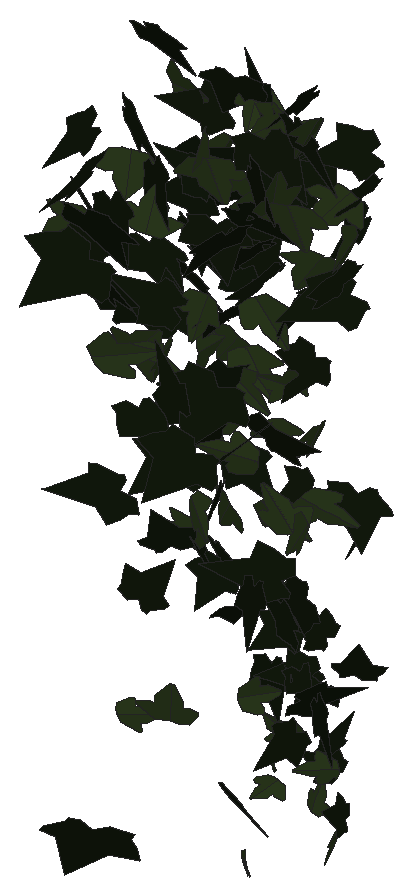
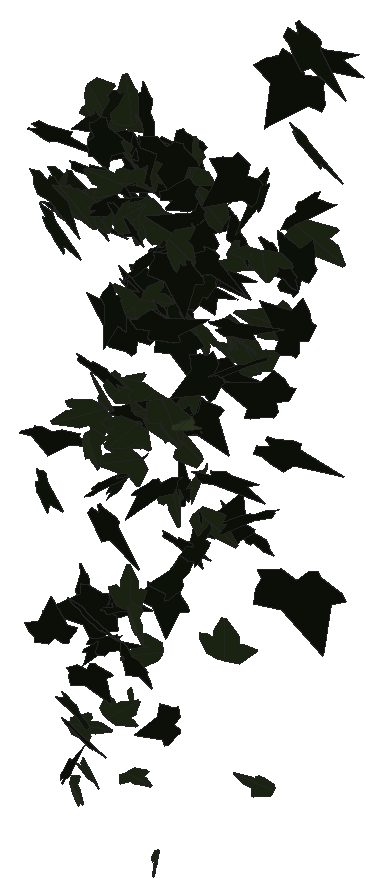
# SketchUp Ruby script. Lengths in inches.
U = 1.inch
M = Sketchup.active_model
def pt(a) = Geom::Point3d.new(a.map { |v| v * U })
def face(e, loops, mat)
  f = e.add_face(loops[0].map { |a| pt(a) })
  loops[1..].each { |l| e.add_face(l.map { |a| pt(a) }).erase! }
  f.material = f.back_material = mat if mat
  f
end
# faces: each face lists its corners as indices into pts; further lists are holes
def faces(e, pts, list, mat = nil) = list.each { |f| face(e, (f[0].is_a?(Array) ? f : [f]).map { |l| l.map { |i| pts[i] } }, mat) }
# xy, xz, yz: faces in a plane at the given z, y or x. An outline is a flat list of corners, or four numbers for a rectangle; further outlines are holes
def ring(l) = l.size == 4 ? [[l[0], l[1]], [l[2], l[1]], [l[2], l[3]], [l[0], l[3]]] : l.each_slice(2).to_a
def flat(e, list, mat, &to3) = list.each { |f| face(e, (f[0].is_a?(Array) ? f : [f]).map { |l| ring(l).map { |u, v| to3.(u, v) } }, mat) }
def xy(e, z, list, mat = nil) = flat(e, list, mat) { |x, y| [x, y, z] }
def xz(e, y, list, mat = nil) = flat(e, list, mat) { |x, z| [x, y, z] }
def yz(e, x, list, mat = nil) = flat(e, list, mat) { |y, z| [x, y, z] }
def lines(e, pts, list) = list.each { |a, b| e.add_line(pt(pts[a]), pt(pts[b])) }
# prism: a flat outline (further loops are holes) pulled along v
def prism(e, loops, v, mat = nil)
  f = face(e, loops, mat); d = Geom::Vector3d.new(v.map { |x| x * U })
  f.pushpull(f.normal.samedirection?(d) ? d.length : -d.length)
end
def box(e, o, s, mat = nil) = prism(e, [[o, [o[0] + s[0], o[1], o[2]], [o[0] + s[0], o[1] + s[1], o[2]], [o[0], o[1] + s[1], o[2]]]], [0, 0, s[2]], mat)
def at(x, y, z, deg = 0) = Geom::Transformation.translation(pt([x, y, z])) * Geom::Transformation.rotation(ORIGIN, Z_AXIS, deg.degrees)
def axes(o, x, y, z) = Geom::Transformation.new([*x, 0, *y, 0, *z, 0, *pt(o).to_a, 1])
def part(name) = M.definitions.add(name)
# library, detail: a bought-in or finely detailed component or shape, given as its bounding box
def library(name, o, s) = part(name).tap { |d| box(d.entities, o, s) }
def detail(e, o, s) = box(e.add_group.entities, o, s)
def put(e, d, t, mat = nil) = e.add_instance(d, t).tap { |i| i.material = mat if mat }
def group(e, t, mat = nil) = e.add_group.tap { |g| g.transformation = t; g.material = mat if mat }.entities
root = M.entities
M.materials.add("1026 AP 7946 SUNNY SIDE UP").color = [254, 231, 186]
M.materials.add("efeu1").color = [18, 25, 13]
M.materials.add("efeu2").color = [43, 57, 29]
c1 = part("ivyleaf_9")
p = [[1.54,2.16,1.25],[1.36,2.04,1.19],[-0.21,0.99,0.68],[-0.71,1.11,0.82],[-0.85,0.86,0.67],[-0.8,0.17,0.21],
  [-0.9,-0.01,0.1],[-0.67,-0.16,-0.02],[-0.08,-0.08,-0.05],[-0.03,-0.6,-0.4],[0.65,-0.88,-0.66],[0.83,-0.6,-0.49],
  [1.29,-0.42,-0.43],[1.8125,-0.07,-0.26],[1.21,0.44,0.15]]
faces(c1.entities,p,[[0,1,2,3,4,5,6,7,8,9,10,11,12,13,14]],"efeu1")
c2 = part("ivyleaf_10")
p = [[0,0.5,-0.03],[-0.0625,2.02,-0.43],[-0.19,2.01,-0.46],[-0.54,1.05,-0.29],[-0.52,0.625,-0.18],[-0.83,0.76,-0.28],
  [-1.16,0.64,-0.33],[-1.15,0.33,-0.24],[-0.77,-0.39,0.02],[-0.3,-0.51,0.16],[0.04,-0.48,0.23],[-0.02,2.01,-0.4375],
  [-0.06,2.01,-0.43],[0.04,-0.49,0.23],[0.67,-0.49,0.14],[1.38,0.36,-0.2],[1.375,0.51,-0.24],[0.81,0.65,-0.19],
  [0.62,0.59,-0.15],[0.6,1.09,-0.28],[0.5,1.23,-0.31]]
faces(c2.entities,p,[[0,1,2,3,4,5,6,7,8,9,10],[11,12,0,13,14,15,16,17,18,19,20]],"efeu2")
put(root,c1,axes([142.13,203.52,266.92],[-0.59838,-0.25995,0.14465],[-0.15209,-0.10927,-0.47412],[0.44014,-0.39117,0.03283]),"1026 AP 7946 SUNNY SIDE UP")
put(root,c1,axes([142.22,203.6,254.35],[0.33655,0.29324,-0.32482],[-0.26346,-0.26965,-0.37513],[-0.62578,0.27124,-0.01675]),"1026 AP 7946 SUNNY SIDE UP")
put(root,c1,axes([141.34,204.61,268.11],[-0.41422,0.33967,-0.1751],[0.1295,-0.15324,-0.44287],[-0.58443,-0.27471,0.02597]),"1026 AP 7946 SUNNY SIDE UP")
put(root,c1,axes([141.35,204.56,267.15],[0.68349,0.0532,-0.11463],[-0.16482,-0.05756,-0.4493],[-0.10301,0.44506,-0.04172]),"1026 AP 7946 SUNNY SIDE UP")
put(root,c1,axes([143.26,205.375,262.24],[-0.60942,-0.18272,0.00796],[0.01229,-0.03707,-0.44],[0.28737,-0.3859,0.03571]),"1026 AP 7946 SUNNY SIDE UP")
put(root,c1,axes([144.04,206.29,259.13],[-0.33232,0.03705,-0.34007],[0.49382,-0.10596,-0.21987],[-0.17119,-0.37756,0.02593]),"1026 AP 7946 SUNNY SIDE UP")
put(root,c1,axes([139.9,206.48,265.28],[0.05679,-0.12956,-0.36457],[0.20893,-0.3275,0.13586],[-0.55334,-0.13696,0.01388]),"1026 AP 7946 SUNNY SIDE UP")
put(root,c1,axes([142.28,206.16,262.59],[-0.1674,-0.29108,0.27585],[0.11646,0.25946,0.32045],[-0.61269,0.12885,-0.01446]),"1026 AP 7946 SUNNY SIDE UP")
put(root,c1,axes([143.36,206.1,261.8],[-0.12627,0.36421,-0.14879],[-0.03686,0.14481,0.38499],[0.61618,0.0833,-0.00746]),"1026 AP 7946 SUNNY SIDE UP")
put(root,c1,axes([142.68,206.83,262.8],[-0.60903,-0.22483,-0.08626],[0.14251,0.00751,-0.45963],[0.34854,-0.39594,0.0372]),"1026 AP 7946 SUNNY SIDE UP")
put(root,c1,axes([140.22,206.88,259.71],[-0.09943,-0.11542,-0.35875],[-0.37918,-0.25236,0.13005],[-0.43344,0.24724,-0.03147]),"1026 AP 7946 SUNNY SIDE UP")
put(root,c1,axes([144.11,206.95,259.09],[-0.30554,-0.0104,0.33923],[-0.50482,-0.08012,-0.19822],[0.11666,-0.37391,0.03075]),"1026 AP 7946 SUNNY SIDE UP")
put(root,c1,axes([139.48,206.94,267.4],[-0.51522,0.16645,-0.14793],[0.16639,-0.10839,-0.37636],[-0.30408,-0.34133,0.0447]),"1026 AP 7946 SUNNY SIDE UP")
put(root,c2,axes([139.25,207.05,265.23],[-0.35022,-0.11625,0.30223],[-0.35381,-0.19439,-0.25591],[0.34927,-0.31349,0.04382]),"1026 AP 7946 SUNNY SIDE UP")
put(root,c2,axes([140.03,206.78,262.63],[-0.15968,-0.07963,0.36959],[0.3595,0.2783,0.13178],[-0.45328,0.24878,-0.02569]),"1026 AP 7946 SUNNY SIDE UP")
put(root,c1,axes([142.73,207.02,266.11],[-0.15301,0.33929,-0.26201],[0.07773,-0.25207,-0.36464],[-0.66403,-0.10769,0.01768]),"1026 AP 7946 SUNNY SIDE UP")
put(root,c1,axes([140.64,207.07,257.44],[-0.27102,0.20408,0.21536],[0.24627,-0.13876,0.27329],[0.38624,0.23168,-0.02313]),"1026 AP 7946 SUNNY SIDE UP")
put(root,c2,axes([141.07,207.46,254.83],[-0.50153,-0.12449,-0.00868],[-0.02899,0.02609,0.35143],[-0.19397,0.31798,-0.03007]),"1026 AP 7946 SUNNY SIDE UP")
put(root,c1,axes([143.97,207.52,257.72],[0.01058,-0.34074,0.11709],[0.00193,0.11563,0.35176],[-0.56577,-0.00598,0.00339]),"1026 AP 7946 SUNNY SIDE UP")
put(root,c2,axes([143.51,207.62,266.85],[-0.14274,-0.37927,-0.07801],[-0.0417,-0.06928,0.40123],[-0.60604,0.09409,-0.00923]),"1026 AP 7946 SUNNY SIDE UP")
put(root,c1,axes([143.3,207.67,261.59],[0.06292,-0.11241,0.37205],[0.44095,-0.23581,-0.10882],[0.40052,0.27728,0.06135]),"1026 AP 7946 SUNNY SIDE UP")
put(root,c2,axes([140.82,207.61,262.67],[0.12967,-0.3648,-0.01894],[-0.01585,0.01445,-0.38515],[0.57397,0.08281,-0.00635]),"1026 AP 7946 SUNNY SIDE UP")
put(root,c1,axes([143.78,207.85,255.18],[-0.01763,-0.03729,-0.36455],[0.20536,-0.32953,0.0296],[-0.52009,-0.12885,0.02405]),"1026 AP 7946 SUNNY SIDE UP")
put(root,c1,axes([142.82,207.79,267.21],[0.06414,-0.06484,-0.39952],[0.59443,-0.09942,0.05756],[-0.16793,-0.37669,0.05115]),"1026 AP 7946 SUNNY SIDE UP")
put(root,c2,axes([143.94,207.61,266.78],[-0.57044,-0.11345,-0.0675],[0.11788,-0.02386,-0.38903],[0.16833,-0.36776,0.0437]),"1026 AP 7946 SUNNY SIDE UP")
put(root,c1,axes([138.63,208.02,264.84],[0.07673,-0.20187,0.41712],[0.18726,-0.38834,-0.21592],[0.68798,0.12822,0.01225]),"1026 AP 7946 SUNNY SIDE UP")
put(root,c2,axes([140.13,207.8,262.27],[-0.05549,-0.01653,-0.3496],[0.4883,-0.13976,-0.02708],[-0.21638,-0.31115,0.02855]),"1026 AP 7946 SUNNY SIDE UP")
put(root,c1,axes([143.13,207.6875,264.95],[-0.24728,0.38585,-0.01038],[-0.01578,-0.01733,-0.42904],[-0.60682,-0.15679,0.01539]),"1026 AP 7946 SUNNY SIDE UP")
put(root,c2,axes([139.96,207.85,262.29],[-0.47982,-0.06192,0.15725],[0.22931,0.04941,0.32055],[-0.12152,0.33776,-0.01598]),"1026 AP 7946 SUNNY SIDE UP")
put(root,c1,axes([138.6,208.12,263.45],[0.20155,-0.20763,0.37149],[0.25656,-0.32337,-0.25263],[0.60364,0.20677,-0.01666]),"1026 AP 7946 SUNNY SIDE UP")
put(root,c1,axes([139.13,208.07,265.125],[-0.23987,-0.03836,-0.3583],[0.5497,-0.00751,-0.15725],[0.01336,-0.37951,0.03709]),"1026 AP 7946 SUNNY SIDE UP")
put(root,c2,axes([143.88,207.95,259.69],[0.29643,-0.30327,-0.08176],[-0.07717,0.06088,-0.36739],[0.48616,0.19458,-0.00846]),"1026 AP 7946 SUNNY SIDE UP")
put(root,c1,axes([140.55,208.09,258.125],[0.28484,0.08872,0.25547],[-0.37665,-0.06815,0.2054],[0.17036,-0.29902,0.02699]),"1026 AP 7946 SUNNY SIDE UP")
put(root,c2,axes([141.25,208.01,259.23],[-0.0883,0.33883,0.04532],[-0.02443,0.04005,-0.35348],[-0.53632,-0.05761,0.00864]),"1026 AP 7946 SUNNY SIDE UP")
put(root,c1,axes([144.01,208.32,255.64],[-0.08166,-0.01533,-0.39435],[0.5788,-0.10871,-0.04761],[-0.1664,-0.3706,0.02792]),"1026 AP 7946 SUNNY SIDE UP")
put(root,c1,axes([141.25,208.21,260.82],[-0.05853,0.23373,-0.25671],[0.02904,-0.25025,-0.24483],[-0.53794,-0.03894,0.01472]),"1026 AP 7946 SUNNY SIDE UP")
put(root,c1,axes([141.89,208.17,253.11],[0.39149,-0.16311,0.04338],[0.03946,-0.04005,-0.30621],[0.2623,0.24947,-0.01868]),"1026 AP 7946 SUNNY SIDE UP")
put(root,c1,axes([142.41,208.04,266.1],[0.54405,0.09283,0.09657],[0.15538,-0.01027,-0.36741],[-0.13654,0.35818,-0.03332]),"1026 AP 7946 SUNNY SIDE UP")
put(root,c2,axes([143.37,208.1875,259.53],[0.44804,0.07573,0.20431],[-0.31486,-0.01218,0.30176],[0.10892,-0.3467,0.0319]),"1026 AP 7946 SUNNY SIDE UP")
put(root,c1,axes([140.37,208.33,263.17],[-0.32606,-0.20416,-0.17098],[-0.21293,-0.09665,0.29831],[-0.35338,0.24662,-0.02198]),"1026 AP 7946 SUNNY SIDE UP")
put(root,c2,axes([141.09,208.46,267.04],[-0.06813,0.16566,-0.30754],[-0.01053,-0.30221,-0.173],[-0.53803,-0.01506,0.04233]),"1026 AP 7946 SUNNY SIDE UP")
put(root,c1,axes([141.51,208.44,257.74],[-0.45217,-0.04754,-0.10807],[0.16951,-0.01388,-0.29881],[0.06262,-0.30569,0.02854]),"1026 AP 7946 SUNNY SIDE UP")
put(root,c2,axes([140.91,208.35,258.43],[-0.24914,-0.0192,0.27815],[-0.4065,-0.08239,-0.16275],[0.12668,-0.30212,0.0248]),"1026 AP 7946 SUNNY SIDE UP")
put(root,c2,axes([142.13,208.44,260.41],[0.0036,0.03782,0.3531],[-0.48914,-0.14717,0.01802],[0.23317,-0.30931,0.03235]),"1026 AP 7946 SUNNY SIDE UP")
put(root,c1,axes([144.61,208.25,265.18],[-0.30351,0.37172,0.0393],[-0.07983,0.01407,-0.42959],[-0.58179,-0.19585,0.03845]),"1026 AP 7946 SUNNY SIDE UP")
put(root,c2,axes([139.84,208.29,264.83],[0.44649,0.1982,-0.10615],[0.09931,0.0905,0.35529],[0.33777,-0.2886,0.03585]),"1026 AP 7946 SUNNY SIDE UP")
put(root,c1,axes([140.42,208.61,259.73],[-0.56399,-0.13094,0.05247],[-0.05681,-0.0511,-0.39198],[0.21394,-0.35877,0.03426]),"1026 AP 7946 SUNNY SIDE UP")
put(root,c1,axes([144.47,208.61,264.73],[-0.63382,-0.03907,0.09414],[-0.13126,-0.07575,-0.41212],[0.08541,-0.40637,0.06529]),"1026 AP 7946 SUNNY SIDE UP")
put(root,c2,axes([141.28,208.43,266.53],[-0.54369,-0.18316,-0.08286],[0.14254,-0.00259,-0.40058],[0.27966,-0.35476,0.04308]),"1026 AP 7946 SUNNY SIDE UP")
put(root,c1,axes([141.27,208.53,258.97],[0.03668,0.20271,0.24666],[-0.12288,-0.22759,0.20601],[0.47631,-0.07432,0.03415]),"1026 AP 7946 SUNNY SIDE UP")
put(root,c1,axes([139.71,208.66,265.8125],[-0.14746,-0.01813,-0.38421],[0.57634,-0.0773,-0.09156],[-0.11119,-0.37661,0.03499]),"1026 AP 7946 SUNNY SIDE UP")
put(root,c2,axes([143.77,208.4375,260.01],[-0.25443,-0.11091,-0.30979],[0.45648,0.0904,-0.19516],[0.21138,-0.32872,0.04857]),"1026 AP 7946 SUNNY SIDE UP")
put(root,c1,axes([139.24,208.46,266.98],[0.41531,-0.21474,-0.24183],[-0.30938,0.12749,-0.34929],[0.39132,0.3287,-0.01949]),"1026 AP 7946 SUNNY SIDE UP")
put(root,c2,axes([143.73,208.65,265.2],[-0.38701,-0.21539,0.15319],[-0.14334,-0.12258,-0.3363],[0.38695,-0.26083,0.02864]),"1026 AP 7946 SUNNY SIDE UP")
put(root,c2,axes([140.85,208.69,263.24],[0.52504,-0.16914,0.03698],[0.03354,-0.03927,-0.38495],[0.27012,0.33363,-0.02409]),"1026 AP 7946 SUNNY SIDE UP")
put(root,c1,axes([140.6875,208.64,258.12],[0.43114,-0.24511,-0.09537],[-0.13525,0.04024,-0.37766],[0.38834,0.28614,-0.02565]),"1026 AP 7946 SUNNY SIDE UP")
put(root,c2,axes([142.6,208.66,259.38],[-0.32619,0.01013,-0.28697],[0.42819,-0.06712,-0.21178],[-0.09402,-0.34082,0.0311]),"1026 AP 7946 SUNNY SIDE UP")
put(root,c1,axes([143.45,208.59,257.71],[0.024,-0.02601,-0.38442],[-0.58645,-0.0276,-0.0139],[-0.04181,0.37229,-0.02568]),"1026 AP 7946 SUNNY SIDE UP")
put(root,c2,axes([141.57,208.66,259.02],[-0.36426,0.14355,0.20412],[-0.29439,0.06994,-0.27844],[-0.24608,-0.29616,0.03095]),"1026 AP 7946 SUNNY SIDE UP")
put(root,c1,axes([142.63,209.07,266.1],[-0.22773,-0.21111,0.28057],[-0.18168,-0.24994,-0.2632],[0.51205,-0.18257,0.03139]),"1026 AP 7946 SUNNY SIDE UP")
put(root,c1,axes([141.08,208.86,264.93],[-0.27977,-0.23134,-0.19605],[0.22292,0.12823,-0.29845],[0.41344,-0.22568,0.02826]),"1026 AP 7946 SUNNY SIDE UP")
put(root,c2,axes([143.4,208.89,267.96],[-0.01035,-0.33417,0.11126],[-0.00626,-0.10984,-0.34497],[0.5531,-0.0075,-0.00182]),"1026 AP 7946 SUNNY SIDE UP")
put(root,c1,axes([140.6,208.97,265.82],[-0.04066,-0.34119,-0.01525],[-0.00547,-0.01264,0.35241],[-0.53683,0.02597,-0.00243]),"1026 AP 7946 SUNNY SIDE UP")
put(root,c2,axes([138.91,208.88,265.65],[0.54423,0.13229,-0.00426],[0.01062,-0.03132,-0.38051],[-0.20789,0.34473,-0.0306]),"1026 AP 7946 SUNNY SIDE UP")
put(root,c1,axes([142.29,208.86,267.22],[-0.1201,-0.25737,-0.29935],[0.26288,0.24385,-0.26771],[0.54895,-0.17308,0.06271]),"1026 AP 7946 SUNNY SIDE UP")
put(root,c1,axes([140.32,209.15,264.31],[0.03429,-0.2502,0.28769],[0.05261,-0.27874,-0.26028],[0.58888,0.03947,0.0065]),"1026 AP 7946 SUNNY SIDE UP")
put(root,c1,axes([143.4375,208.58,255.49],[0.04481,0.24141,-0.29325],[-0.00017,0.28686,0.25109],[0.58852,-0.0183,0.0224]),"1026 AP 7946 SUNNY SIDE UP")
put(root,c2,axes([142.01,208.67,255.01],[-0.00973,-0.00463,0.32185],[0.07578,0.30875,0.0075],[-0.48546,0.04829,-0.00528]),"1026 AP 7946 SUNNY SIDE UP")
put(root,c1,axes([142.91,209.03,267.69],[0.35432,-0.36658,0.01932],[-0.00764,-0.02742,-0.44304],[0.57729,0.22463,-0.01772]),"1026 AP 7946 SUNNY SIDE UP")
put(root,c1,axes([140.09,208.87,262.4],[-0.55136,-0.01566,0.07396],[0.10995,0.03782,0.36012],[-0.03593,0.35594,-0.0329]),"1026 AP 7946 SUNNY SIDE UP")
put(root,c2,axes([142.01,209.02,263.42],[0.42972,0.04242,0.2566],[0.39137,0.01583,-0.2843],[-0.06614,0.36927,-0.0151]),"1026 AP 7946 SUNNY SIDE UP")
put(root,c2,axes([140.625,209.11,260.43],[0.22366,-0.11455,-0.33538],[0.44381,-0.16279,0.18548],[-0.3106,-0.31511,0.02352]),"1026 AP 7946 SUNNY SIDE UP")
put(root,c1,axes([141.14,208.95,263.01],[-0.01218,0.32028,-0.11176],[0.00391,-0.11027,-0.33069],[-0.53262,-0.00813,0.00013]),"1026 AP 7946 SUNNY SIDE UP")
put(root,c2,axes([142.45,208.86,253.8],[-0.04774,0.08133,0.28033],[-0.2767,0.20883,-0.08345],[-0.34963,-0.17637,0.02776]),"1026 AP 7946 SUNNY SIDE UP")
put(root,c1,axes([141.45,208.92,256.6875],[0.12001,0.2845,-0.0232],[0.00137,-0.02522,-0.30351],[-0.44896,0.07597,-0.00713]),"1026 AP 7946 SUNNY SIDE UP")
put(root,c2,axes([143.96,209.35,265.41],[0.06003,-0.08873,0.38543],[0.22311,-0.34674,-0.10153],[0.56277,0.14693,-0.00087]),"1026 AP 7946 SUNNY SIDE UP")
put(root,c2,axes([142.01,209.12,265.79],[-0.29896,-0.31855,-0.03717],[0.05925,0.01734,-0.38131],[0.50028,-0.19241,0.02295]),"1026 AP 7946 SUNNY SIDE UP")
put(root,c1,axes([138.62,208.91,262.27],[-0.00831,0.03444,0.39447],[0.5491,0.16014,-0.00894],[-0.25213,0.34764,-0.03248]),"1026 AP 7946 SUNNY SIDE UP")
put(root,c1,axes([140.42,209.18,265.33],[-0.01987,-0.04755,-0.36037],[-0.52241,-0.11593,0.02794],[-0.1864,0.32999,-0.0399]),"1026 AP 7946 SUNNY SIDE UP")
put(root,c1,axes([142.39,209.4375,256.31],[-0.29398,-0.15325,0.14812],[-0.14848,-0.11195,-0.24858],[0.29624,-0.2082,0.0224]),"1026 AP 7946 SUNNY SIDE UP")
put(root,c2,axes([138.59,209.2,253.22],[0.12049,-0.02499,-0.23886],[0.36578,0.02315,0.07681],[0.02246,-0.24296,0.03044]),"1026 AP 7946 SUNNY SIDE UP")
put(root,c1,axes([140.71,209.39,257.52],[0.31388,-0.27413,0.07524],[0.04444,-0.07156,-0.34923],[0.4445,0.20073,-0.01822]),"1026 AP 7946 SUNNY SIDE UP")
put(root,c1,axes([140.83,209.08,261.27],[0.05366,0.03754,0.34863],[0.44855,0.18215,-0.04941],[-0.2917,0.287,-0.01186]),"1026 AP 7946 SUNNY SIDE UP")
put(root,c1,axes([144.09,209.42,259.84],[-0.30108,-0.25414,-0.15768],[0.18671,0.09943,-0.3256],[0.42622,-0.22308,0.03125]),"1026 AP 7946 SUNNY SIDE UP")
put(root,c1,axes([140.12,209.13,265.87],[0.1257,0.04792,0.3873],[0.55013,0.13766,-0.09398],[-0.228,0.35857,-0.01324]),"1026 AP 7946 SUNNY SIDE UP")
put(root,c2,axes([140.52,209.1,261.96],[0.02725,-0.0465,-0.34816],[0.11097,0.33129,-0.04133],[0.52439,-0.06769,0.02684]),"1026 AP 7946 SUNNY SIDE UP")
put(root,c2,axes([141.17,209.42,265.83],[-0.3904,-0.07011,0.2606],[-0.3618,-0.11058,-0.26446],[0.19991,-0.33706,0.03029]),"1026 AP 7946 SUNNY SIDE UP")
put(root,c1,axes([141.9,209.51,255.29],[-0.2843,-0.03128,-0.30027],[0.46063,-0.01503,-0.18575],[0.00575,-0.34252,0.03355]),"1026 AP 7946 SUNNY SIDE UP")
put(root,c2,axes([142.25,209.58,261.55],[-0.13496,-0.11238,-0.27387],[-0.26605,-0.20427,0.14439],[-0.36652,0.18966,-0.00397]),"1026 AP 7946 SUNNY SIDE UP")
put(root,c1,axes([141.54,209.29,264.43],[0.03195,0.32467,-0.07917],[-0.00744,-0.07855,-0.33559],[-0.52524,0.02086,-0.00006]),"1026 AP 7946 SUNNY SIDE UP")
put(root,c2,axes([141.08,209.46,261.3],[0.23695,0.02622,0.31429],[0.48122,-0.01565,-0.15452],[0.00389,0.33977,-0.02937]),"1026 AP 7946 SUNNY SIDE UP")
put(root,c2,axes([142.03,209.39,260.65],[-0.42066,-0.06566,-0.16391],[0.25354,0.00529,-0.28219],[0.09312,-0.31103,0.0279]),"1026 AP 7946 SUNNY SIDE UP")
put(root,c1,axes([142.62,209.17,263.43],[-0.0713,0.0014,-0.40462],[-0.42762,0.28516,0.03506],[0.44561,0.27388,-0.0311]),"1026 AP 7946 SUNNY SIDE UP")
put(root,c1,axes([138.7,209.49,259.79],[0.07226,-0.32268,-0.16969],[0.09011,0.16862,-0.32649],[0.56117,0.01447,0.07427]),"1026 AP 7946 SUNNY SIDE UP")
put(root,c1,axes([142.74,209.64,255.33],[-0.26659,-0.06096,0.23447],[-0.31379,-0.11272,-0.18463],[0.19796,-0.26077,0.02311]),"1026 AP 7946 SUNNY SIDE UP")
put(root,c1,axes([142.64,209.51,255.38],[0.05084,-0.23142,-0.15291],[-0.0251,0.14629,-0.23983],[0.43045,0.03586,0.00408]),"1026 AP 7946 SUNNY SIDE UP")
put(root,c1,axes([141.54,209.8,264.84],[-0.16019,-0.14956,0.31096],[-0.23244,-0.2645,-0.18743],[0.4773,-0.17901,0.01309]),"1026 AP 7946 SUNNY SIDE UP")
put(root,c2,axes([142.03,209.5,267.34],[0.34347,-0.21334,-0.18901],[-0.24398,0.10061,-0.31231],[0.36762,0.2661,-0.03068]),"1026 AP 7946 SUNNY SIDE UP")
put(root,c1,axes([142.8,209.72,266.71],[-0.59173,-0.10881,-0.03608],[0.07117,-0.0335,-0.40114],[0.16473,-0.3764,0.04372]),"1026 AP 7946 SUNNY SIDE UP")
put(root,c2,axes([142.3,209.61,253.84],[-0.2849,-0.05715,-0.19515],[-0.29221,-0.03776,0.19496],[-0.1054,0.25916,-0.013]),"1026 AP 7946 SUNNY SIDE UP")
put(root,c1,axes([138.84,209.64,263.4],[0.08224,-0.38915,-0.11404],[0.10359,0.11614,-0.39579],[0.62673,0.03187,0.08038]),"1026 AP 7946 SUNNY SIDE UP")
put(root,c1,axes([141.19,209.49,259.65],[0.09954,-0.25996,-0.26012],[-0.06592,0.24784,-0.27385],[0.56438,0.07479,0.01389]),"1026 AP 7946 SUNNY SIDE UP")
put(root,c1,axes([142.57,209.77,265.86],[-0.21586,-0.06243,0.28095],[-0.31749,-0.18871,-0.15012],[0.30527,-0.24041,0.04252]),"1026 AP 7946 SUNNY SIDE UP")
put(root,c2,axes([141.84,209.68,256.76],[-0.14052,-0.31249,-0.10768],[-0.03236,-0.10095,0.33414],[-0.51622,0.09139,0.00836]),"1026 AP 7946 SUNNY SIDE UP")
put(root,c2,axes([141.81,209.66,252.6],[0.20967,0.07895,-0.15796],[-0.18523,-0.10064,-0.15904],[-0.19893,0.17692,-0.0184]),"1026 AP 7946 SUNNY SIDE UP")
put(root,c2,axes([141.25,209.5,250.79],[-0.16511,0.15597,0.08143],[-0.08551,0.05741,-0.19297],[-0.26064,-0.11764,0.01172]),"1026 AP 7946 SUNNY SIDE UP")
put(root,c2,axes([143.125,209.75,253.34],[-0.04852,0.0046,0.26755],[-0.21626,-0.22212,-0.01409],[0.34643,-0.13802,0.02868]),"1026 AP 7946 SUNNY SIDE UP")
put(root,c2,axes([141.28,209.61,261.82],[0.45707,0.08167,0.1889],[0.28551,0.02867,-0.31031],[-0.13299,0.34224,-0.01696]),"1026 AP 7946 SUNNY SIDE UP")
put(root,c1,axes([140.46,209.87,266.86],[-0.19721,-0.03322,0.37913],[-0.49369,-0.19572,-0.12951],[0.30693,-0.33616,0.03529]),"1026 AP 7946 SUNNY SIDE UP")
put(root,c1,axes([142.55,209.88,259.25],[-0.20052,-0.14154,0.23732],[-0.1752,-0.20552,-0.19416],[0.38854,-0.16572,0.03493]),"1026 AP 7946 SUNNY SIDE UP")
put(root,c1,axes([140.91,209.6,267.8],[0.34688,0.15561,-0.23112],[-0.25389,-0.15963,-0.27747],[-0.34762,0.27187,-0.02797]),"1026 AP 7946 SUNNY SIDE UP")
put(root,c2,axes([143.24,209.77,251.85],[0.14687,-0.21188,0.1121],[0.06311,-0.10252,-0.23911],[0.37006,0.10158,-0.00371]),"1026 AP 7946 SUNNY SIDE UP")
put(root,c1,axes([144.06,209.77,267.22],[-0.48172,0.01567,0.16118],[-0.24709,-0.0269,-0.31455],[-0.00263,-0.3429,0.03002]),"1026 AP 7946 SUNNY SIDE UP")
put(root,c1,axes([141.15,209.77,263.47],[-0.07659,0.03562,0.33655],[-0.5144,-0.03432,-0.04663],[0.04546,-0.32831,0.03942]),"1026 AP 7946 SUNNY SIDE UP")
put(root,c1,axes([141.45,209.57,263.97],[-0.34789,0.23087,0.1569],[0.19525,-0.08949,0.32789],[0.38734,0.25247,-0.02436]),"1026 AP 7946 SUNNY SIDE UP")
put(root,c2,axes([141.16,209.95,264.29],[0.13524,0.14235,-0.32325],[-0.2036,-0.28724,-0.17205],[-0.50331,0.15444,-0.01726]),"1026 AP 7946 SUNNY SIDE UP")
put(root,c1,axes([142.64,209.86,262.15],[-0.51042,-0.01769,-0.12209],[0.18754,-0.01807,-0.33417],[0.01635,-0.34506,0.02173]),"1026 AP 7946 SUNNY SIDE UP")
put(root,c2,axes([143.38,209.8125,265.96],[0.55952,-0.06529,-0.15333],[-0.23965,-0.0122,-0.37086],[0.08721,0.38537,-0.0354]),"1026 AP 7946 SUNNY SIDE UP")
put(root,c2,axes([141.76,210.03,265.99],[-0.02652,0.06698,0.32538],[0.06355,-0.31296,0.06885],[0.50309,0.04306,0.00846]),"1026 AP 7946 SUNNY SIDE UP")
put(root,c1,axes([143.3,209.98,252.21],[-0.0535,0.00882,0.27305],[-0.18722,-0.23922,-0.00895],[0.37251,-0.11897,0.03472]),"1026 AP 7946 SUNNY SIDE UP")
put(root,c2,axes([139.26,209.94,266.9],[-0.21669,0.05038,0.37635],[0.54923,-0.1063,0.15034],[0.1846,0.37542,-0.00552]),"1026 AP 7946 SUNNY SIDE UP")
put(root,c1,axes([142.39,210.08,267.76],[-0.25399,0.00302,-0.3081],[0.23824,-0.29225,-0.08905],[-0.4055,-0.17359,0.14066]),"1026 AP 7946 SUNNY SIDE UP")
put(root,c2,axes([140.28,210.08,265.9375],[0.02752,-0.29563,0.25253],[0.0782,-0.24326,-0.30523],[0.60048,0.04523,0.02817]),"1026 AP 7946 SUNNY SIDE UP")
put(root,c1,axes([139.49,209.85,263.03],[0.51421,-0.14313,-0.00841],[-0.03105,-0.02687,-0.36638],[0.2232,0.326,-0.0316]),"1026 AP 7946 SUNNY SIDE UP")
put(root,c1,axes([141.75,210,266.05],[-0.30952,-0.02151,-0.26461],[0.40457,-0.03291,-0.20058],[-0.02069,-0.32183,0.03629]),"1026 AP 7946 SUNNY SIDE UP")
put(root,c1,axes([138.66,209.8,268.01],[0.57306,-0.01867,-0.01242],[-0.02113,-0.02949,-0.37483],[0.02773,0.36345,-0.0289]),"1026 AP 7946 SUNNY SIDE UP")
put(root,c2,axes([141.16,210,267.36],[0.26352,0.26121,-0.12868],[-0.08138,-0.11671,-0.31986],[-0.44897,0.17447,-0.01755]),"1026 AP 7946 SUNNY SIDE UP")
put(root,c2,axes([142.66,209.91,252.32],[0.33399,-0.14105,0.01305],[0.00329,0.0274,0.26167],[-0.22277,-0.21107,0.02344]),"1026 AP 7946 SUNNY SIDE UP")
put(root,c2,axes([142.11,210.05,261.52],[0.19965,-0.17863,-0.19766],[0.22046,-0.13253,0.22311],[-0.3469,-0.18703,0.02803]),"1026 AP 7946 SUNNY SIDE UP")
put(root,c1,axes([142.71,209.98,254.9],[0.12382,0.09556,-0.21711],[-0.17846,-0.1787,-0.12789],[-0.31797,0.13751,-0.01277]),"1026 AP 7946 SUNNY SIDE UP")
put(root,c1,axes([143.875,210.08,259.01],[-0.27235,0.11917,-0.23762],[0.2674,-0.15851,-0.21622],[-0.30972,-0.24164,0.02228]),"1026 AP 7946 SUNNY SIDE UP")
put(root,c1,axes([142.93,209.85,256.15],[-0.18521,0.1702,0.20853],[-0.2246,0.1443,-0.21079],[-0.34859,-0.1834,0.02502]),"1026 AP 7946 SUNNY SIDE UP")
put(root,c2,axes([141.47,210.03,256.7],[0.14416,-0.30861,0.02186],[-0.00099,-0.02414,-0.33171],[0.4866,0.09138,-0.00715]),"1026 AP 7946 SUNNY SIDE UP")
put(root,c2,axes([140.7,209.94,261.83],[-0.46058,0.034,0.19156],[-0.29535,-0.01722,-0.302],[-0.03052,-0.34642,0.03177]),"1026 AP 7946 SUNNY SIDE UP")
put(root,c1,axes([140.4,209.9,265.33],[0.36073,0.07561,-0.25853],[-0.36695,-0.09415,-0.24912],[-0.18903,0.32705,-0.00977]),"1026 AP 7946 SUNNY SIDE UP")
put(root,c1,axes([143.12,209.87,253.25],[-0.15493,0.16148,0.19483],[-0.20429,0.13888,-0.19202],[-0.33213,-0.16075,0.02723]),"1026 AP 7946 SUNNY SIDE UP")
put(root,c1,axes([141.44,209.84,267.31],[0.07377,-0.08708,0.34707],[-0.12507,0.32877,0.10073],[-0.53344,-0.08913,0.02438]),"1026 AP 7946 SUNNY SIDE UP")
put(root,c1,axes([143.54,210.05,255.47],[0.33965,0.09727,0.13617],[-0.2163,-0.01018,0.24026],[0.13944,-0.25275,0.04103]),"1026 AP 7946 SUNNY SIDE UP")
put(root,c2,axes([142.57,210.07,260.47],[0.00821,-0.29945,0.03227],[0.00535,-0.03297,-0.30872],[0.47368,0.00556,0.00293]),"1026 AP 7946 SUNNY SIDE UP")
put(root,c1,axes([143.04,209.87,253.74],[-0.21493,0.23878,-0.01438],[-0.00176,0.01701,0.28344],[0.37623,0.13649,-0.00689]),"1026 AP 7946 SUNNY SIDE UP")
put(root,c2,axes([140.03,210.1875,261.72],[-0.30332,-0.00514,0.07627],[0.05111,-0.19123,0.07242],[0.10495,0.07827,0.18515]),"1026 AP 7946 SUNNY SIDE UP")
put(root,c1,axes([143.61,210.16,265.41],[-0.4286,0.14641,-0.22209],[0.26018,-0.14531,-0.31682],[-0.31797,-0.31625,0.04012]),"1026 AP 7946 SUNNY SIDE UP")
put(root,c2,axes([142,209.84,266.71],[0.23952,0.11869,-0.30454],[0.32156,0.21577,0.19862],[0.38533,-0.25384,0.02356]),"1026 AP 7946 SUNNY SIDE UP")
put(root,c1,axes([143.79,209.9,266.11],[-0.20725,0.352,0.05764],[-0.07239,0.0402,-0.38585],[-0.55525,-0.13663,0.02879]),"1026 AP 7946 SUNNY SIDE UP")
